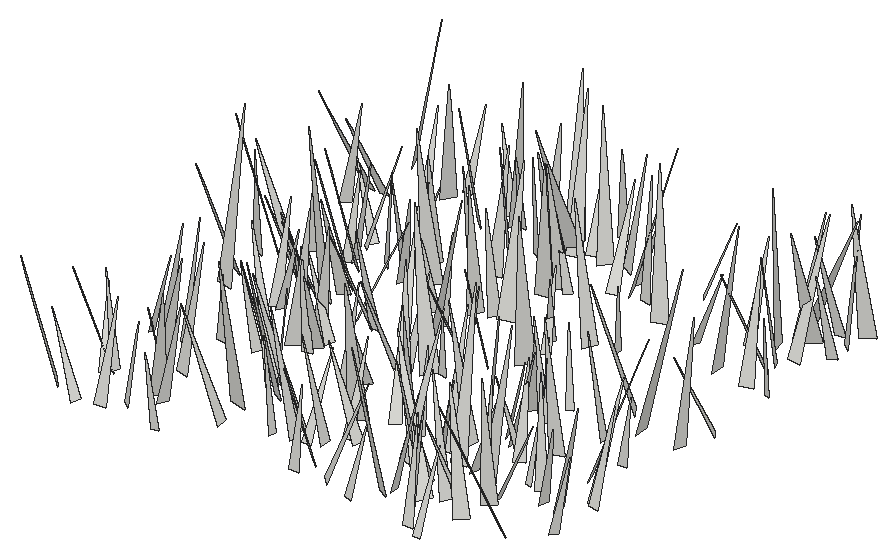
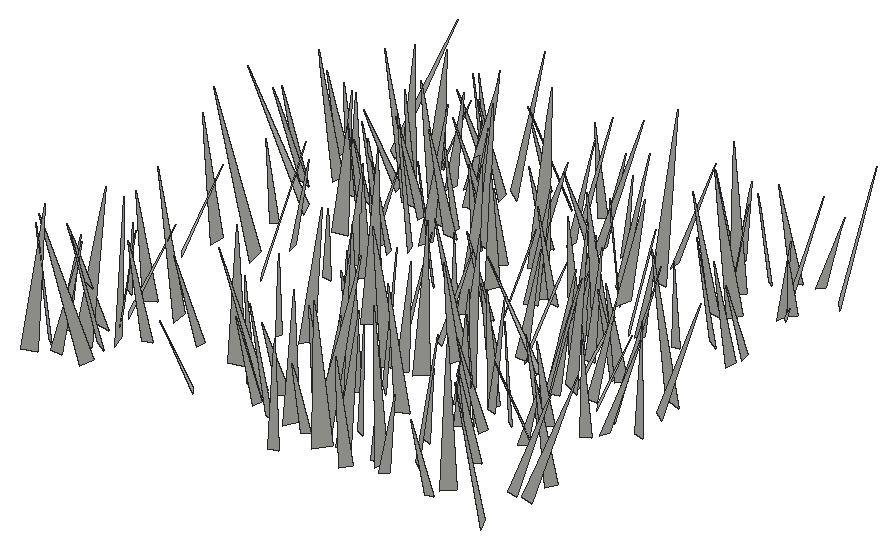
# SketchUp Ruby script. Lengths in inches.
U = 1.inch
M = Sketchup.active_model
def pt(a) = Geom::Point3d.new(a.map { |v| v * U })
def face(e, loops, mat)
  f = e.add_face(loops[0].map { |a| pt(a) })
  loops[1..].each { |l| e.add_face(l.map { |a| pt(a) }).erase! }
  f.material = f.back_material = mat if mat
  f
end
# faces: each face lists its corners as indices into pts; further lists are holes
def faces(e, pts, list, mat = nil) = list.each { |f| face(e, (f[0].is_a?(Array) ? f : [f]).map { |l| l.map { |i| pts[i] } }, mat) }
# xy, xz, yz: faces in a plane at the given z, y or x. An outline is a flat list of corners, or four numbers for a rectangle; further outlines are holes
def ring(l) = l.size == 4 ? [[l[0], l[1]], [l[2], l[1]], [l[2], l[3]], [l[0], l[3]]] : l.each_slice(2).to_a
def flat(e, list, mat, &to3) = list.each { |f| face(e, (f[0].is_a?(Array) ? f : [f]).map { |l| ring(l).map { |u, v| to3.(u, v) } }, mat) }
def xy(e, z, list, mat = nil) = flat(e, list, mat) { |x, y| [x, y, z] }
def xz(e, y, list, mat = nil) = flat(e, list, mat) { |x, z| [x, y, z] }
def yz(e, x, list, mat = nil) = flat(e, list, mat) { |y, z| [x, y, z] }
def lines(e, pts, list) = list.each { |a, b| e.add_line(pt(pts[a]), pt(pts[b])) }
# prism: a flat outline (further loops are holes) pulled along v
def prism(e, loops, v, mat = nil)
  f = face(e, loops, mat); d = Geom::Vector3d.new(v.map { |x| x * U })
  f.pushpull(f.normal.samedirection?(d) ? d.length : -d.length)
end
def box(e, o, s, mat = nil) = prism(e, [[o, [o[0] + s[0], o[1], o[2]], [o[0] + s[0], o[1] + s[1], o[2]], [o[0], o[1] + s[1], o[2]]]], [0, 0, s[2]], mat)
def at(x, y, z, deg = 0) = Geom::Transformation.translation(pt([x, y, z])) * Geom::Transformation.rotation(ORIGIN, Z_AXIS, deg.degrees)
def axes(o, x, y, z) = Geom::Transformation.new([*x, 0, *y, 0, *z, 0, *pt(o).to_a, 1])
def part(name) = M.definitions.add(name)
# library, detail: a bought-in or finely detailed component or shape, given as its bounding box
def library(name, o, s) = part(name).tap { |d| box(d.entities, o, s) }
def detail(e, o, s) = box(e.add_group.entities, o, s)
def put(e, d, t, mat = nil) = e.add_instance(d, t).tap { |i| i.material = mat if mat }
def group(e, t, mat = nil) = e.add_group.tap { |g| g.transformation = t; g.material = mat if mat }.entities
root = M.entities
c1 = part("fur_instance\#9")
p = [[0.8125,0,1.79],[0.67,-0.02,1.48],[0,-0.11,0],[0,0.11,0]]
faces(c1.entities,p,[[0,1,2,3]])
put(root,c1,axes([499.51,133.05,-21.66],[-3.13069,-4.74867,0.6646],[-4.79451,3.11096,-0.35688],[0.06511,0.75154,5.67659]))
put(root,c1,axes([499.34,151.17,-21.66],[-1.38983,-5.84462,0.0201],[-5.82782,1.38425,-0.46046],[-0.44334,0.12603,5.98992]))
put(root,c1,axes([499.54,108.77,-21.66],[-4.76298,-4.61729,1.21885],[-4.61962,4.89113,0.47635],[1.20999,0.49843,6.61653]))
put(root,c1,axes([498.79,136.74,-21.66],[-1.48378,-4.80354,1.85374],[-5.06695,1.70492,0.36217],[0.91449,1.65264,5.01442]))
put(root,c1,axes([501.26,138.23,-21.66],[-5.40823,0.65228,0.52882],[0.69912,5.40686,0.48075],[0.46513,-0.5426,5.42617]))
put(root,c1,axes([499.18,148.04,-21.66],[4.20018,-2.603,1.54886],[-2.85846,-4.28223,0.55487],[-1.0019,1.30501,4.91012]))
put(root,c1,axes([500.125,130.58,-21.66],[2.12447,7.8086,2.15105],[8.03257,-2.31646,0.47574],[-1.03873,-1.94278,8.07844]))
put(root,c1,axes([500.91,151.1875,-21.66],[-0.25255,-4.7231,0.0991],[-4.68784,0.23828,-0.59045],[-0.58449,0.12972,4.69284]))
put(root,c1,axes([499.63,156.77,-21.66],[6.18065,2.99725,1.89028],[2.99834,-6.44896,0.42186],[-1.88855,-0.42956,6.85609]))
put(root,c1,axes([502.44,135.65,-21.66],[-5.20648,-5.71637,1.32602],[-5.85189,5.18966,-0.6046],[0.43665,1.3904,7.70836]))
put(root,c1,axes([501.52,112.53,-21.66],[-2.57238,2.98987,0.10946],[2.97729,2.57237,-0.29516],[0.29502,0.10983,3.93311]))
put(root,c1,axes([500.25,120.59,-21.66],[3.57631,0.31891,0.97988],[0.16002,-3.66803,0.60973],[-1.01797,0.54376,3.53835]))
put(root,c1,axes([501.83,113.28,-21.66],[-3.65311,-4.50937,0.62916],[-4.48426,3.70309,0.50402],[0.78847,0.16789,5.78149]))
put(root,c1,axes([500.41,122.3,-21.66],[4.80103,-0.44543,1.50068],[-0.59366,-4.99749,0.41591],[-1.44845,0.57184,4.80368]))
put(root,c1,axes([502.05,113.41,-21.66],[-4.36363,0.98227,0.81119],[0.91976,4.432,-0.41906],[0.88144,0.23814,4.45315]))
put(root,c1,axes([502.77,107.23,-21.66],[-3.82314,1.91513,0.41484],[1.95484,3.79049,0.51675],[0.13566,-0.64863,4.24466]))
put(root,c1,axes([502.1875,139.66,-21.66],[2.0816,-3.74764,1.04429],[-3.88491,-2.06538,0.3318],[-0.20701,1.076,4.27408]))
put(root,c1,axes([504.64,135.04,-21.66],[-3.58425,-2.16039,0.18109],[-2.16614,3.55434,-0.47063],[-0.08907,0.49634,4.15845]))
put(root,c1,axes([503.76,120.56,-21.66],[2.58353,5.00263,1.49189],[5.09313,-2.78069,0.50442],[-1.14546,-1.08079,5.60772]))
put(root,c1,axes([505.53,144,-21.66],[-3.05082,2.35934,0.28628],[2.37608,3.01778,0.45074],[-0.05159,-0.53147,3.83025]))
put(root,c1,axes([504.86,107.9,-21.66],[-0.99114,4.85366,1.48422],[5.00835,1.18049,-0.51592],[0.82303,-1.33855,4.92689]))
put(root,c1,axes([505.76,134.44,-21.66],[0.4513,-4.46287,0.47479],[-4.46772,-0.49211,-0.3789],[-0.42669,0.43236,4.4696]))
put(root,c1,axes([507.15,139.75,-21.66],[2.82941,3.82153,3.56935],[4.50896,-3.83832,0.53527],[-2.64833,-2.45217,4.72474]))
put(root,c1,axes([505.79,130.4,-21.66],[-2.49427,4.27012,1.59064],[4.35584,2.76683,-0.59729],[1.33819,-1.04698,4.90903]))
put(root,c1,axes([505.79,140.12,-21.66],[2.7326,-2.75522,2.01665],[-3.2693,-2.85632,0.52755],[-0.98478,1.83723,3.84448]))
put(root,c1,axes([505.4,143.0625,-21.66],[2.99735,3.72962,0.28981],[3.68324,-3.00724,0.60693],[-0.65404,0.15682,4.74613]))
put(root,c1,axes([506.6875,148.98,-21.66],[-1.85743,4.94831,0.92273],[4.99711,1.93095,-0.29602],[0.60509,-0.75691,5.27714]))
put(root,c1,axes([506.23,155.69,-21.66],[-0.0874,4.08723,0.80677],[4.1529,0.14964,-0.30818],[0.33125,-0.79758,4.07653]))
put(root,c1,axes([505.91,122.86,-21.66],[0.58274,-3.68979,0.92218],[-3.78198,-0.46356,0.53511],[0.40205,0.98748,3.697]))
put(root,c1,axes([506.19,140.71,-21.66],[4.45017,0.43948,1.54669],[0.28501,-4.6951,0.51402],[-1.58245,0.39027,4.44218]))
put(root,c1,axes([505.49,154.04,-21.66],[5.14782,-4.26055,1.16689],[-4.27581,-5.25589,-0.32723],[-1.10966,0.4872,6.67423]))
put(root,c1,axes([508.16,133.28,-21.66],[-3.2308,-2.41105,0.08917],[-2.40238,3.20101,-0.49122],[-0.22293,0.4467,4.00124]))
put(root,c1,axes([505.3,115.69,-21.66],[5.59181,-3.37862,1.09906],[-3.46581,-5.63815,0.30113],[-0.78177,0.82912,6.52631]))
put(root,c1,axes([506.53,109.35,-21.66],[2.33806,3.32528,1.40975],[3.5899,-2.32407,-0.47188],[-0.3968,-1.43269,4.03749]))
put(root,c1,axes([506.39,130.38,-21.66],[3.89931,-1.45547,0.98195],[-1.58431,-3.9476,0.44006],[-0.75669,0.76505,4.13877]))
put(root,c1,axes([506.81,116.46,-21.66],[1.78136,5.8506,1.71123],[6.09225,-1.76893,-0.29408],[-0.20572,-1.72409,6.10871]))
put(root,c1,axes([508.73,136.93,-21.66],[-4.07714,-4.72232,1.18622],[-4.85623,4.056,-0.54439],[0.3528,1.25658,6.21506]))
put(root,c1,axes([507.76,113.27,-21.66],[-3.40624,-2.616,1.08161],[-2.59295,3.56228,0.44999],[1.13575,0.28715,4.27123]))
put(root,c1,axes([508.3125,133.97,-21.66],[-2.90002,-7.26429,3.03178],[-7.85451,2.88308,-0.60516],[0.51793,3.0479,7.79832]))
put(root,c1,axes([509.41,123.39,-21.66],[-3.58724,1.8714,1.40372],[2.1412,3.66165,0.59026],[0.94225,-1.19623,4.00275]))
put(root,c1,axes([508.99,135.62,-21.66],[1.67149,-5.33301,0.8085],[-5.34441,-1.75188,-0.5067],[-0.72935,0.6152,5.5658]))
put(root,c1,axes([508.61,141.82,-21.66],[2.85129,3.39796,1.84964],[3.79237,-2.9092,-0.50161],[-0.76499,-1.75715,4.40731]))
put(root,c1,axes([507.59,112.29,-21.66],[3.73697,-5.4189,0.58942],[-5.45085,-3.71358,0.41766],[0.01126,0.72231,6.56925]))
put(root,c1,axes([508.7,111.6,-21.66],[4.80209,-1.99507,1.20954],[-2.10711,-4.89697,0.2883],[-1.00169,0.73669,5.19204]))
put(root,c1,axes([510.51,123.42,-21.66],[-3.88391,-3.01754,1.00768],[-2.99103,4.00531,0.46572],[1.08383,0.24005,4.89626]))
put(root,c1,axes([510.35,152.18,-21.66],[-3.95359,-4.39819,1.62013],[-4.4402,4.19331,0.54823],[1.50116,0.81969,5.8885]))
put(root,c1,axes([510.1,129.22,-21.66],[0.02895,-4.95019,0.58964],[-4.94989,0.0415,0.59139],[0.59214,0.58889,4.91483]))
put(root,c1,axes([511.05,107.54,-21.66],[0.17752,-3.57602,1.3313],[-3.7929,-0.31113,-0.32997],[-0.41733,1.30655,3.56518]))
put(root,c1,axes([511.69,155,-21.66],[-3.05036,2.77962,1.08054],[2.93347,3.07501,0.37088],[0.53722,-1.00823,4.11016]))
put(root,c1,axes([509.55,144.25,-21.66],[4.16125,-1.09144,0.28201],[-1.11074,-4.15389,0.31328],[-0.19241,0.37504,4.29058]))
put(root,c1,axes([511.19,141.1,-21.66],[-1.65824,-4.82946,1.36253],[-4.95542,1.80194,0.35604],[0.78993,1.16588,5.09379]))
put(root,c1,axes([510.92,143.82,-21.66],[4.15437,2.45212,1.76514],[2.75663,-4.30471,-0.50784],[-1.23677,-1.35794,4.79727]))
put(root,c1,axes([514.11,119.74,-21.66],[-6.63605,2.7216,0.19643],[2.70208,6.62626,-0.52374],[0.38006,0.41041,7.15332]))
put(root,c1,axes([512.28,148.49,-21.66],[0.90627,3.33198,1.59944],[3.57947,-1.20149,0.47479],[-0.9207,-1.39138,3.42023]))
put(root,c1,axes([513.33,128.29,-21.66],[-4.0044,1.49429,0.5536],[1.5481,4.00291,0.3933],[0.37782,-0.56428,4.25599]))
put(root,c1,axes([511.1,126.29,-21.66],[5.02607,-4.57327,2.19343],[-4.92834,-5.13329,0.59007],[-1.19892,1.92923,6.76964]))
put(root,c1,axes([511.59,144.67,-21.66],[4.45698,-3.93649,1.376],[-3.92382,-4.64074,-0.56675],[-1.41173,0.47074,5.91941]))
put(root,c1,axes([512.8125,125.92,-21.66],[-0.34045,4.62028,2.07312],[5.05885,0.21591,0.34957],[-0.23002,-2.08976,4.6196]))
put(root,c1,axes([511.52,140.38,-21.66],[4.68677,-2.0034,0.66372],[-1.95488,-4.73014,-0.47351],[-0.79535,-0.17932,5.07496]))
put(root,c1,axes([511.71,128.9375,-21.66],[3.13383,-5.16211,1.39491],[-5.34355,-3.08346,0.59403],[-0.19921,1.50298,6.00961]))
put(root,c1,axes([514.76,111.93,-21.66],[-5.6933,-0.47947,0.5538],[-0.44449,5.71072,0.37467],[0.58224,-0.32872,5.70116]))
put(root,c1,axes([514.36,132.65,-21.66],[-3.87512,-3.17972,0.32504],[-3.163,3.88842,0.32938],[0.4601,-0.04943,5.00187]))
put(root,c1,axes([512.65,154.14,-21.66],[7.01983,-0.71592,2.31882],[-0.6287,-7.39114,-0.37866],[-2.34397,-0.1616,7.04608]))
put(root,c1,axes([513,127.12,-21.66],[2.62732,-3.98087,0.28129],[-3.95197,-2.64215,-0.47983],[-0.55532,-0.03119,4.74551]))
put(root,c1,axes([513.67,141.65,-21.66],[3.74176,-6.61768,2.63887],[-6.89022,-4.11933,-0.5604],[-1.81167,1.99888,7.58159]))
put(root,c1,axes([513.51,153.95,-21.66],[0.0585,-4.06465,0.78718],[-4.11626,0.02739,0.44734],[0.44434,0.78888,4.04038]))
put(root,c1,axes([513.92,115.11,-21.66],[-1.04012,-7.65192,1.88155],[-7.84849,1.17518,0.4406],[0.70237,1.80029,7.70971]))
put(root,c1,axes([514.86,132.5,-21.66],[-0.19276,-5.01478,1.27598],[-5.16585,0.1124,-0.33865],[-0.30027,1.28555,5.00705]))
put(root,c1,axes([512.35,133.34,-21.66],[4.96423,2.67259,0.04648],[2.6631,-4.93667,-0.5706],[0.22978,-0.52435,5.60898]))
put(root,c1,axes([515.69,118.32,-21.66],[-3.47477,-5.64058,1.59223],[-5.83486,3.50381,-0.32112],[0.55295,1.52727,6.61718]))
put(root,c1,axes([514.34,119.94,-21.66],[3.53151,3.08583,1.68165],[3.37882,-3.63698,-0.42174],[-0.96639,-1.43941,4.67077]))
put(root,c1,axes([514.82,156.24,-21.66],[3.66382,-3.28739,1.57998],[-3.52995,-3.75957,0.36325],[-0.918,1.33625,4.90903]))
put(root,c1,axes([517.04,133.63,-21.66],[-2.44616,4.11048,0.29857],[4.09909,2.46258,-0.31948],[0.42742,-0.0923,4.7726]))
put(root,c1,axes([516.91,138.1,-21.66],[1.11597,-3.30458,1.27259],[-3.40234,-1.37051,-0.57526],[-0.98175,0.99326,3.44016]))
put(root,c1,axes([516.94,146.01,-21.66],[-1.46748,5.77462,2.34569],[6.13429,1.76496,-0.50731],[1.10405,-2.13089,5.93652]))
put(root,c1,axes([517.49,150.93,-21.66],[-2.05605,-4.2865,1.82271],[-4.5186,2.31917,0.35698],[1.13077,1.47345,4.74068]))
put(root,c1,axes([516.99,153.87,-21.66],[3.45501,-4.88886,0.26504],[-4.85303,-3.46254,-0.60598],[-0.64754,-0.13474,5.95575]))
put(root,c1,axes([518.46,154.87,-21.66],[-5.59489,5.13542,2.2708],[5.22691,5.9344,-0.54239],[2.05147,-1.11455,7.57503]))
put(root,c1,axes([519.33,113.08,-21.66],[-4.34694,-0.07841,1.0456],[-0.20123,4.43859,-0.5037],[1.02905,0.53671,4.31837]))
put(root,c1,axes([520.95,114.79,-21.66],[-7.49054,-0.65717,0.9559],[-0.61994,7.54719,0.33069],[0.98046,-0.24861,7.51203]))
put(root,c1,axes([518.55,123.625,-21.66],[0.78552,4.64999,1.51438],[4.88897,-0.70993,-0.35606],[0.11721,-1.55126,4.70241]))
put(root,c1,axes([520.07,128.59,-21.66],[-3.91317,-2.34388,0.53173],[-2.28614,3.94348,0.55853],[0.74167,-0.21123,4.52711]))
put(root,c1,axes([520.09,152.82,-21.66],[-1.2461,7.24945,1.28302],[7.36015,1.19663,0.38699],[-0.1701,-1.32928,7.34558]))
put(root,c1,axes([518.94,136.47,-21.66],[-3.54773,2.23846,2.32232],[2.39169,4.14191,-0.33862],[2.16418,-0.90784,4.1812]))
put(root,c1,axes([521.25,113.66,-21.66],[-5.82181,0.2065,0.70872],[0.14567,5.84473,-0.50632],[0.72368,0.48471,5.80343]))
put(root,c1,axes([519.86,123.32,-21.66],[-3.10303,1.40825,1.48641],[1.65077,3.31728,0.3033],[1.21143,-0.91317,3.39411]))
put(root,c1,axes([520.58,143.84,-21.66],[3.92843,5.06138,3.38638],[5.5366,-4.64662,0.52215],[-2.53598,-2.30413,6.38572]))
put(root,c1,axes([519.85,153.3125,-21.66],[2.00321,-7.73932,0.37509],[-7.71802,-2.02729,-0.61059],[-0.68548,0.20889,7.97102]))
put(root,c1,axes([519.69,139.96,-21.66],[-4.92901,3.2655,3.81824],[4.17297,5.6397,0.56365],[2.798,-2.65855,5.88565]))
put(root,c1,axes([519.32,134.93,-21.66],[6.35559,1.23086,1.81432],[1.1106,-6.60444,0.5901],[-1.89033,0.25813,6.44673]))
put(root,c1,axes([520.04,124.77,-21.66],[2.51881,-4.55482,0.15905],[-4.51842,-2.51942,-0.59372],[-0.59628,-0.14918,5.17091]))
put(root,c1,axes([521.14,153.76,-21.66],[-1.57636,3.66287,0.67143],[3.67727,1.64614,-0.34684],[0.58749,-0.47537,3.97256]))
put(root,c1,axes([521.26,140.54,-21.66],[-4.23654,2.45749,2.21286],[2.8358,4.54981,0.37637],[1.70124,-1.46429,4.88322]))
put(root,c1,axes([521.87,134.79,-21.66],[-2.1706,-3.79382,0.07549],[-3.76138,2.16267,0.53397],[0.50075,-0.20018,4.33814]))
put(root,c1,axes([521.2,128.93,-21.66],[0.22863,4.55848,1.01522],[4.65358,-0.13679,-0.43379],[0.39321,-1.03161,4.54355]))
put(root,c1,axes([521.46,157.78,-21.66],[0.51611,-4.80053,1.29544],[-4.96034,-0.40702,0.46794],[0.34389,1.33374,4.80546]))
put(root,c1,axes([523.23,129.39,-21.66],[-5.88987,4.84378,2.23578],[5.14185,6.04195,0.45575],[1.42207,-1.78441,7.61217]))
put(root,c1,axes([523.01,153.36,-21.66],[-6.12251,3.37612,2.03098],[3.42132,6.417,-0.35327],[1.95387,-0.65732,6.98272]))
put(root,c1,axes([522.54,140.6,-21.66],[-2.30774,6.81626,2.09214],[7.04491,2.51871,-0.43516],[1.09893,-1.8327,7.18315]))
put(root,c1,axes([522.52,113.63,-21.66],[-0.04754,4.40868,0.34675],[4.41199,0.07095,-0.29716],[0.30179,-0.34273,4.39891]))
put(root,c1,axes([522.82,147.74,-21.66],[2.11565,-6.08651,1.80009],[-6.2822,-2.27872,-0.32139],[-0.90548,1.58863,6.43571]))
put(root,c1,axes([523.81,114.625,-21.66],[-5.16901,0.01394,1.37798],[0.15537,5.32107,0.52899],[1.36927,-0.55116,5.14189]))
put(root,c1,axes([523.72,147.47,-21.66],[1.42768,-3.34431,1.65268],[-3.54003,-1.77266,-0.52903],[-1.17641,1.27565,3.59761]))
put(root,c1,axes([522.42,145.85,-21.66],[2.16747,-6.96935,1.82134],[-7.20329,-2.08612,0.58967],[0.04123,1.91397,7.27476]))
put(root,c1,axes([524.3,124.68,-21.66],[-5.32179,3.05618,1.70346],[3.04909,5.5718,-0.47069],[1.71611,-0.42222,6.11884]))
put(root,c1,axes([523.41,119.57,-21.66],[4.47344,-6.57845,1.38646],[-6.62258,-4.59864,-0.45163],[-1.15746,0.88686,7.94253]))
put(root,c1,axes([525.99,116.33,-21.66],[-4.59292,1.38597,0.57425],[1.45174,4.5724,0.57548],[0.37836,-0.71958,4.76284]))
put(root,c1,axes([525.14,111.48,-21.66],[-3.21192,-3.98216,0.77509],[-3.98629,3.28152,0.34045],[0.75355,0.38579,5.10471]))
put(root,c1,axes([524.18,129.88,-21.66],[-0.14412,-3.47359,1.04669],[-3.58722,0.2928,0.47779],[0.54152,1.01518,3.44359]))
put(root,c1,axes([524.84,116.37,-21.66],[-1.136,4.49998,0.83575],[4.53043,1.22799,-0.4539],[0.65076,-0.69355,4.61891]))
put(root,c1,axes([524.62,109.34,-21.66],[-0.53957,3.97433,2.02364],[4.38519,0.84425,-0.48882],[0.81275,-1.91664,3.98089]))
put(root,c1,axes([526.11,133.62,-21.66],[-3.38614,-3.10021,1.02366],[-3.22386,3.40798,-0.34286],[0.51569,0.94841,4.57818]))
put(root,c1,axes([526.26,120.94,-21.66],[-3.1637,4.01487,0.30871],[3.99884,3.17867,-0.35895],[0.47305,-0.01931,5.09895]))
put(root,c1,axes([525.09,153.69,-21.66],[2.3418,4.95634,1.60959],[5.19702,-2.35112,-0.32146],[-0.38351,-1.59595,5.4723]))
put(root,c1,axes([526.66,149.78,-21.66],[-2.17484,4.53028,0.06229],[4.50087,2.16823,-0.54601],[0.51907,0.1805,4.99552]))
put(root,c1,axes([528.7,138.19,-21.66],[-2.71022,2.78687,0.60598],[2.7235,2.77712,-0.59105],[0.8464,-0.01233,3.84222]))
put(root,c1,axes([527.74,140.09,-21.66],[3.24769,-2.54753,0.32293],[-2.51539,-3.26077,-0.4265],[-0.51676,-0.13836,4.10555]))
put(root,c1,axes([527.39,152.45,-21.66],[3.65064,-1.60023,0.53489],[-1.66152,-3.63138,0.47591],[-0.29361,0.65299,3.95745]))
put(root,c1,axes([528.51,135.75,-21.66],[5.1556,-5.75467,2.21602],[-5.90961,-5.43588,-0.36737],[-1.76168,1.39363,7.71761]))
put(root,c1,axes([528.6875,127.21,-21.66],[4.00395,3.96639,1.91354],[4.25291,-4.1539,-0.28869],[-1.14309,-1.56151,5.62855]))
put(root,c1,axes([527.8,109.65,-21.66],[3.6626,3.70148,0.35684],[3.71844,-3.64024,-0.40601],[0.03906,-0.53912,5.19141]))
put(root,c1,axes([527.76,150.89,-21.66],[6.78168,2.91502,1.19431],[2.8839,-6.88568,0.43057],[-1.26762,-0.07012,7.36906]))
put(root,c1,axes([529.3,120.5,-21.66],[-3.40994,2.09099,1.78678],[2.1335,3.80705,-0.3836],[1.73581,-0.57158,3.98156]))
put(root,c1,axes([529.69,150.39,-21.66],[1.56528,5.39191,1.82425],[5.61252,-1.77733,0.43748],[-0.9488,-1.61836,5.59744]))
put(root,c1,axes([529.52,119.41,-21.66],[1.75829,5.41715,3.42251],[6.36736,-1.87488,-0.30363],[-0.71818,-3.36006,5.68726]))
put(root,c1,axes([530.79,141.53,-21.66],[-6.02179,2.8816,2.13168],[3.11245,6.27078,0.31555],[1.77772,-1.21792,6.66828]))
put(root,c1,axes([530.97,116.43,-21.66],[1.53253,6.73152,0.42824],[6.72346,-1.5597,0.45586],[-0.5402,-0.31526,6.8887]))
put(root,c1,axes([531.11,108.48,-21.66],[1.148,3.43718,0.90942],[3.54891,-1.0498,-0.51218],[0.21566,-1.0212,3.58745]))
put(root,c1,axes([532.92,110.96,-21.66],[-3.69542,-5.95234,1.80806],[-6.20183,3.68953,-0.52934],[0.48649,1.82006,6.98615]))
put(root,c1,axes([532.63,119.9,-21.66],[-0.26987,6.47949,0.83868],[6.52839,0.23411,0.29205],[-0.25936,-0.84936,6.47853]))
put(root,c1,axes([532.91,148.32,-21.66],[-2.11891,6.73628,2.3501],[7.12334,2.13432,0.30482],[0.39806,-2.33612,7.05509]))
put(root,c1,axes([533.54,122.05,-21.66],[-6.59669,1.20746,2.1658],[1.44471,6.87425,0.5679],[2.0153,-0.97558,6.6822]))
put(root,c1,axes([533.3,142.1875,-21.66],[3.51099,-0.42801,1.09439],[-0.295,-3.65871,-0.48452],[-1.13748,-0.37227,3.50364]))
put(root,c1,axes([536.25,112.23,-21.66],[-6.04879,4.39479,0.23194],[4.40071,6.03643,0.38865],[-0.04117,-0.45072,7.46666]))
put(root,c1,axes([533.01,118.72,-21.66],[4.24569,0.44069,0.96407],[0.53821,-4.32495,-0.39327],[-0.91322,-0.50013,4.25034]))
put(root,c1,axes([533.04,154.1,-21.66],[3.15167,2.15202,0.19961],[2.1362,-3.1554,0.29004],[-0.32814,0.12762,3.80527]))
put(root,c1,axes([534.81,113.94,-21.66],[-5.38028,-3.08502,1.66928],[-3.07413,5.61908,0.47644],[1.68926,0.39986,6.18367]))
put(root,c1,axes([533.375,111.98,-21.66],[4.7353,0.6555,1.15241],[0.55235,-4.8611,0.49538],[-1.20525,0.34759,4.75472]))
put(root,c1,axes([534.83,118.82,-21.66],[-0.16365,8.04006,1.71484],[8.20749,0.06185,0.49328],[-0.46944,-1.72152,8.02659]))
put(root,c1,axes([533.94,123.73,-21.66],[5.56182,2.46032,2.03104],[2.73268,-5.78042,-0.48104],[-1.64644,-1.28288,6.06264]))
put(root,c1,axes([534.6,115.11,-21.66],[1.52104,-3.59534,0.18519],[-3.58042,-1.53172,-0.32978],[-0.37596,0.04131,3.88989]))
put(root,c1,axes([533.81,129.92,-21.66],[3.85722,-2.97975,0.1804],[-2.96484,-3.85827,-0.33622],[-0.3481,-0.15623,4.86251]))
put(root,c1,axes([536.03,128.91,-21.66],[-4.24357,2.27798,1.78244],[2.54082,4.44811,0.36434],[1.38223,-1.18292,4.80254]))
put(root,c1,axes([536.3,131.9375,-21.66],[-0.50007,3.75556,1.02909],[3.87876,0.38868,0.46638],[-0.34425,-1.07612,3.75989]))
put(root,c1,axes([534.99,125.27,-21.66],[3.94564,1.0984,0.79467],[1.2,-3.96752,-0.47419],[-0.63087,-0.67703,4.06813]))
put(root,c1,axes([537.81,113.33,-21.66],[-5.43325,1.77797,0.85582],[1.73658,5.49897,-0.39929],[0.93695,0.1182,5.7028]))
put(root,c1,axes([537.94,123.2,-21.66],[-3.79704,-0.30553,0.54536],[-0.26679,3.82814,0.28712],[0.56533,-0.2455,3.79848]))
put(root,c1,axes([536.48,110.35,-21.66],[-2.09497,-3.98677,2.51489],[-4.46346,2.56262,0.34425],[1.51546,2.03632,4.49052]))
put(root,c1,axes([536.19,124.51,-21.66],[5.46664,-0.56538,0.68203],[-0.51758,-5.49848,-0.40957],[-0.71898,-0.34055,5.48051]))
put(root,c1,axes([538.1875,107.78,-21.66],[0.28645,5.00767,1.03913],[5.08565,-0.389,0.47271],[-0.54104,-1.00525,4.99354]))
put(root,c1,axes([536.61,118.66,-21.66],[4.56446,-0.76979,0.5853],[-0.81155,-4.58493,0.29877],[-0.52586,0.39409,4.61927]))
put(root,c1,axes([539.54,113.39,-21.66],[-4.06839,-1.50308,0.30492],[-1.46625,4.06536,0.47647],[0.44983,-0.34301,4.31092]))
put(root,c1,axes([538.57,122.32,-21.66],[-3.00951,3.51493,1.30262],[3.55292,3.20728,-0.44587],[1.1951,-0.68362,4.60577]))
put(root,c1,axes([537.43,147.52,-21.66],[4.04534,-0.8517,0.30361],[-0.87788,-4.03293,0.38361],[-0.21657,0.43867,4.11619]))
put(root,c1,axes([539.22,123.99,-21.66],[-4.16278,-2.64249,2.71758],[-3.23685,4.57857,-0.50613],[1.97251,1.93665,4.90462]))
put(root,c1,axes([540.73,135.24,-21.66],[-5.52316,-3.7636,0.965],[-3.71814,5.60658,0.58551],[1.12752,0.05244,6.65787]))
put(root,c1,axes([538.85,117.69,-21.66],[1.36969,7.27883,2.41401],[7.66649,-1.2409,-0.6083],[0.18385,-2.48268,7.38156]))
put(root,c1,axes([539.82,106.85,-21.66],[0.7,4.04155,0.09862],[4.02713,-0.70587,0.34334],[-0.35517,-0.03822,4.08733]))
put(root,c1,axes([540.14,115.72,-21.66],[0.9151,5.15761,1.58711],[5.35443,-1.06795,0.38322],[-0.67079,-1.48856,5.22413]))
put(root,c1,axes([540.22,125.26,-21.66],[1.19646,-6.35488,2.45253],[-6.76034,-1.41301,-0.36331],[-0.83491,2.33448,6.45631]))
put(root,c1,axes([540.88,111.62,-21.66],[3.04965,-4.5466,3.26672],[-5.09549,-3.79519,-0.52522],[-2.31926,2.35973,5.44941]))
put(root,c1,axes([541.83,129.61,-21.66],[-4.7779,-0.84592,1.0787],[-0.97294,4.84801,-0.50762],[0.9657,0.69908,4.82558]))
put(root,c1,axes([541.17,115.07,-21.66],[-3.30956,4.62511,3.28339],[5.43338,3.67626,0.29816],[1.62808,-2.86687,5.67942]))
put(root,c1,axes([541.65,119.67,-21.66],[1.21689,3.56799,0.58582],[3.55761,-1.29191,0.47847],[-0.64586,-0.39367,3.73931]))
put(root,c1,axes([541.33,149.89,-21.66],[-0.63443,5.02312,1.44392],[5.17666,0.80438,-0.52377],[0.72032,-1.3566,5.03586]))
put(root,c1,axes([541.2,116.17,-21.66],[3.9948,0.59542,0.26899],[0.55235,-3.96784,0.58004],[-0.34899,0.53573,3.99706]))
put(root,c1,axes([541.73,145.03,-21.66],[7.00703,0.38351,2.14023],[0.30488,-7.32356,0.31416],[-2.15283,0.21111,7.01048]))
put(root,c1,axes([543.16,151.48,-21.66],[-6.66859,-2.01923,2.71074],[-2.32845,7.09045,-0.44648],[2.45024,1.24248,6.95328]))
put(root,c1,axes([543.22,119.51,-21.66],[-1.15441,5.11883,1.74969],[5.40957,1.09949,0.35248],[0.0216,-1.78472,5.23554]))
put(root,c1,axes([545.29,111.8,-21.66],[-4.1792,-5.61615,0.15739],[-5.61189,4.16336,-0.45249],[-0.26934,0.3962,6.98585]))
put(root,c1,axes([545.35,147.34,-21.66],[-3.79986,-3.34827,0.10157],[-3.34083,3.7767,-0.4853],[-0.24505,0.43103,5.04126]))
put(root,c1,axes([545.08,148.8,-21.66],[-4.18009,-2.38384,1.39005],[-2.61185,4.23208,-0.59649],[0.8906,1.22265,4.77494]))
put(root,c1,axes([543.9,152.98,-21.66],[2.83544,5.2975,1.05869],[5.3487,-2.92083,0.29014],[-0.75876,-0.79328,6.00159]))
put(root,c1,axes([543.33,132.85,-21.66],[8.05424,1.38868,1.7961],[1.29513,-8.24767,0.56905],[-1.86468,0.26973,8.15325]))
put(root,c1,axes([545.49,144.27,-21.66],[-2.00411,5.21831,1.67163],[5.38658,2.20263,-0.41796],[1.00489,-1.39973,5.57427]))
put(root,c1,axes([546.15,156.1,-21.66],[0.08099,-5.17118,1.20761],[-5.27072,-0.22549,-0.61212],[-0.64729,1.18913,5.13546]))
put(root,c1,axes([545.11,153.83,-21.66],[3.26606,-6.16963,0.62937],[-6.14796,-3.31446,-0.58694],[-0.81426,0.27855,6.95607]))
put(root,c1,axes([544.66,117.96,-21.66],[4.24921,-1.39082,0.67887],[-1.35455,-4.30166,-0.33452],[-0.74864,-0.11098,4.4585]))
put(root,c1,axes([543.04,155.9,-21.66],[6.75875,-1.16964,0.00047],[-1.16859,-6.75255,0.29358],[0.0496,0.28936,6.85293]))
put(root,c1,axes([545.83,150.24,-21.66],[0.77683,6.56918,0.32302],[6.56801,-0.79193,0.30978],[-0.34589,-0.28401,6.60769]))
put(root,c1,axes([545.76,127.24,-21.66],[0.94774,-3.5048,1.15841],[-3.67796,-0.79512,0.60341],[0.31324,1.26803,3.58018]))
put(root,c1,axes([545.04,123.78,-21.66],[6.72288,3.05704,0.61475],[3.02645,-6.7488,0.46346],[-0.75102,0.16938,7.37074]))
put(root,c1,axes([548.42,136.32,-21.66],[-3.47143,-2.84551,0.09651],[-2.81271,3.45107,0.57956],[0.4415,-0.38766,4.45106]))
put(root,c1,axes([547.79,144.18,-21.66],[1.56672,2.93333,1.48069],[3.11219,-1.85095,0.37383],[-1.05412,-1.105,3.30444]))
put(root,c1,axes([546.27,118,-21.66],[5.73568,-0.06882,1.05766],[0.01363,-5.81521,-0.45231],[-1.05981,-0.44725,5.71823]))
put(root,c1,axes([547.71,155.01,-21.66],[3.73887,4.62596,1.90486],[4.75099,-4.02818,0.45718],[-1.5672,-1.17533,5.9304]))
put(root,c1,axes([548.09,152.66,-21.66],[1.30026,-4.12004,1.09762],[-4.18224,-1.45572,-0.50983],[-0.82967,0.8811,4.29016]))
put(root,c1,axes([547.53,132.71,-21.66],[5.90361,-0.69248,2.28384],[-0.937,-6.27702,0.51884],[-2.19488,0.81708,5.9214]))
put(root,c1,axes([548.19,157.27,-21.66],[-2.64442,5.36733,3.49605],[6.32318,2.79183,0.49668],[1.02376,-3.3795,5.96276]))
put(root,c1,axes([548.03,120.33,-21.66],[1.54833,5.59255,0.52827],[5.59137,-1.58705,0.41342],[-0.54067,-0.39706,5.78818]))
put(root,c1,axes([548.37,120.04,-21.66],[0.17579,4.7582,1.26729],[4.89735,-0.03702,-0.54033],[0.51227,-1.27889,4.73069]))
put(root,c1,axes([548.55,114.46,-21.66],[3.49135,-1.63355,1.08284],[-1.80913,-3.53699,0.49727],[-0.7537,0.9229,3.8224]))
